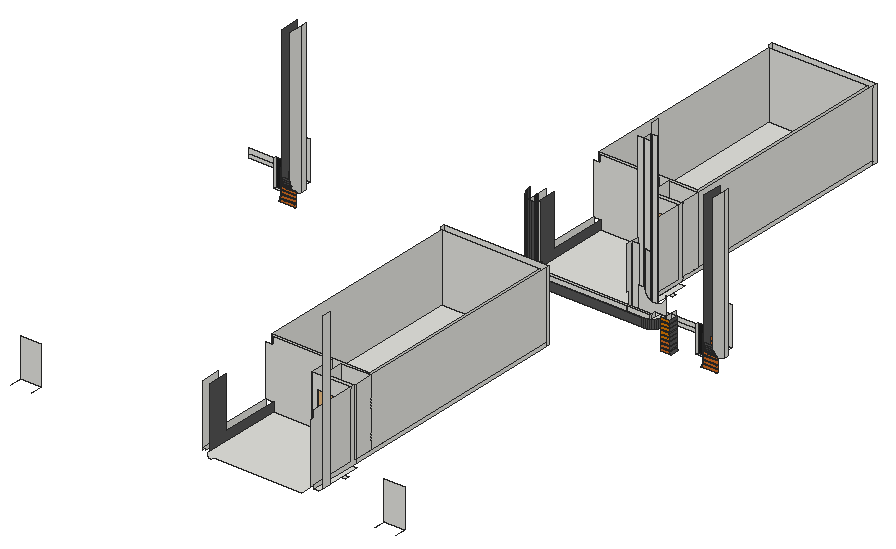
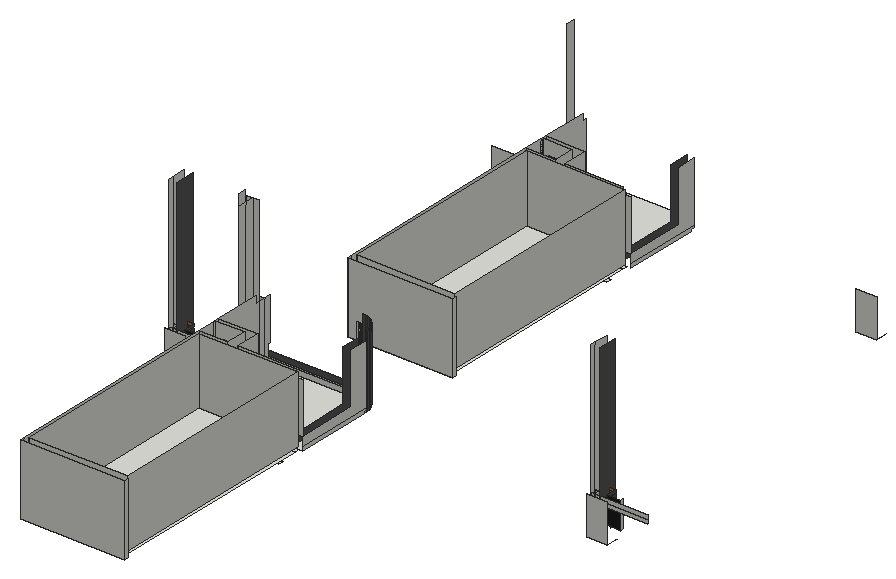
# SketchUp Ruby script. Lengths in inches.
U = 1.inch
M = Sketchup.active_model
def pt(a) = Geom::Point3d.new(a.map { |v| v * U })
def face(e, loops, mat)
  f = e.add_face(loops[0].map { |a| pt(a) })
  loops[1..].each { |l| e.add_face(l.map { |a| pt(a) }).erase! }
  f.material = f.back_material = mat if mat
  f
end
# faces: each face lists its corners as indices into pts; further lists are holes
def faces(e, pts, list, mat = nil) = list.each { |f| face(e, (f[0].is_a?(Array) ? f : [f]).map { |l| l.map { |i| pts[i] } }, mat) }
# xy, xz, yz: faces in a plane at the given z, y or x. An outline is a flat list of corners, or four numbers for a rectangle; further outlines are holes
def ring(l) = l.size == 4 ? [[l[0], l[1]], [l[2], l[1]], [l[2], l[3]], [l[0], l[3]]] : l.each_slice(2).to_a
def flat(e, list, mat, &to3) = list.each { |f| face(e, (f[0].is_a?(Array) ? f : [f]).map { |l| ring(l).map { |u, v| to3.(u, v) } }, mat) }
def xy(e, z, list, mat = nil) = flat(e, list, mat) { |x, y| [x, y, z] }
def xz(e, y, list, mat = nil) = flat(e, list, mat) { |x, z| [x, y, z] }
def yz(e, x, list, mat = nil) = flat(e, list, mat) { |y, z| [x, y, z] }
def lines(e, pts, list) = list.each { |a, b| e.add_line(pt(pts[a]), pt(pts[b])) }
# prism: a flat outline (further loops are holes) pulled along v
def prism(e, loops, v, mat = nil)
  f = face(e, loops, mat); d = Geom::Vector3d.new(v.map { |x| x * U })
  f.pushpull(f.normal.samedirection?(d) ? d.length : -d.length)
end
def box(e, o, s, mat = nil) = prism(e, [[o, [o[0] + s[0], o[1], o[2]], [o[0] + s[0], o[1] + s[1], o[2]], [o[0], o[1] + s[1], o[2]]]], [0, 0, s[2]], mat)
def at(x, y, z, deg = 0) = Geom::Transformation.translation(pt([x, y, z])) * Geom::Transformation.rotation(ORIGIN, Z_AXIS, deg.degrees)
def axes(o, x, y, z) = Geom::Transformation.new([*x, 0, *y, 0, *z, 0, *pt(o).to_a, 1])
def part(name) = M.definitions.add(name)
# library, detail: a bought-in or finely detailed component or shape, given as its bounding box
def library(name, o, s) = part(name).tap { |d| box(d.entities, o, s) }
def detail(e, o, s) = box(e.add_group.entities, o, s)
def put(e, d, t, mat = nil) = e.add_instance(d, t).tap { |i| i.material = mat if mat }
def group(e, t, mat = nil) = e.add_group.tap { |g| g.transformation = t; g.material = mat if mat }.entities
root = M.entities
M.materials.add("[0039_DarkOrange]").color = [219, 120, 0]
M.materials.add("[0041_Chocolate]").color = [210, 105, 30]
M.materials.add("[Color M06]").color = [84, 84, 84]
M.materials.add("[Color M08]").color = [30, 30, 30]
c1 = library("元件\#5",[-4.39,0,0],[5.37,35.83,90.55])
xy(root,90.875,[[1548.19,971.36,1577.46,972.36],[2230.65,971.36,2248.83,972.36],[2302.81,971.36,2332.08,972.36]],"[0041_Chocolate]")
xy(root,95.51,[[1985.87,439.98,2033.5,448.51],[2018.31,1130.875,2065.93,1139.4]])
xy(root,95.83,[[1550.05,971.36,1577.46,972.36],[2230.65,971.36,2246.96,972.36],[2304.68,971.36,2332.08,972.36]],"[0041_Chocolate]")
xy(root,97.27,[[1525.8,986.55,1550.24,991.24],[2280.42,986.55,2304.87,991.24]])
xy(root,97.9375,[[1550.33,971.36,1577.46,972.36],[2230.65,971.36,2246.69,972.36],[2304.96,971.36,2332.08,972.36]],"[0041_Chocolate]")
xy(root,101.1875,[[2078.42,397.86,2125.61,405.05],[2110.86,1088.75,2158.05,1095.9375]])
xy(root,102.89,[[1550.98,971.36,1577.46,972.36],[2230.65,971.36,2246.03,972.36],[2305.61,971.36,2332.08,972.36]],"[0041_Chocolate]")
xy(root,105,[[1550.98,971.36,1577.46,972.36],[2230.65,971.36,2246.03,972.36],[2305.61,971.36,2332.08,972.36]],"[0041_Chocolate]")
xy(root,109.9375,[[1562.99,990,1578.33,993.35],[2317.62,990,2332.96,993.35]])
xy(root,109.95,[[1550.98,971.36,1577.46,972.36],[2230.65,971.36,2246.03,972.36],[2305.61,971.36,2332.08,972.36]],"[0041_Chocolate]")
xy(root,112.0625,[[2230.65,971.36,2246.03,972.36]],"[0039_DarkOrange]")
xy(root,112.0625,[[1550.98,971.36,1577.46,972.36],[2305.61,971.36,2332.08,972.36]],"[0041_Chocolate]")
xy(root,117.02,[[2230.65,971.36,2246.03,972.36]],"[0039_DarkOrange]")
xy(root,117.02,[[1550.98,971.36,1577.46,972.36],[2305.61,971.36,2332.08,972.36]],"[0041_Chocolate]")
xy(root,119.125,[[2230.65,971.36,2246.03,972.36]],"[0039_DarkOrange]")
xy(root,119.125,[[1550.98,971.36,1577.46,972.36],[2305.61,971.36,2332.08,972.36]],"[0041_Chocolate]")
xy(root,124.08,[[2230.65,971.36,2246.03,972.36]],"[0039_DarkOrange]")
xy(root,124.08,[[1550.98,971.36,1577.46,972.36],[2305.61,971.36,2332.08,972.36]],"[0041_Chocolate]")
xy(root,126.125,[[2137,312.8125,2146.71,397.86],[2068.38,397.86,2087.21,397.86,2087.21,448.51,1957.13,448.51,1957.13,439.98,2068.38,439.98],[2087.21,397.86,2137,406.38],[2087.21,406.38,2137,830.91],[1957.13,448.51,2087.21,830.91],
  [1949.9,830.91,2137,838.14],[2012.97,958.64,2008.97,958.91,2005.04,959.6875,2002.6,960.52,2215.38,960.52,2212.34,959.49,2209.17,958.86,2205.95,958.64],[2002.6,960.52,2001.25,960.98,1997.65,962.75,1994.32,964.98,1991.31,967.62,1989.57,969.61,1988.67,970.63,1986.4375,973.96,1984.67,977.56,1983.38,981.35,1982.6,985.28,1982.33,989.28,1982.33,1130.875,2100.82,1130.875,2100.82,1088.75,2169.44,1088.75,2169.44,996.48,2179.15,996.48,2179.15,1003.71,2230.65,1003.71,2230.65,996.48,2230.15,996.48,2230.15,983.34,2230.65,983.34,2230.4375,980.12,2229.81,976.95,2228.77,973.89,2227.34,970.99,2225.54,968.31,2223.41,965.88,2220.98,963.75,2218.3,961.95,2215.4,960.52],[2230.15,983.34,2230.65,993.35],[2230.15,993.35,2230.65,996.48],
  [2169.44,996.48,2179.15,1003.71],[2169.44,1003.71,2179.15,1088.75],[2179.15,1003.71,2179.46,1012.23],[2179.46,1003.71,2181.03,1012.23],[2181.03,1003.71,2190.68,1012.23],
  [2190.68,1003.71,2230.65,1012.23],[2179.15,1012.23,2179.46,1027.17],[2179.46,1012.23,2181.03,1027.17],[2100.82,1088.75,2119.65,1088.75,2119.65,1139.4,1989.57,1139.4,1989.57,1130.875,2100.82,1130.875],[2119.65,1088.75,2169.44,1097.28],
  [2119.65,1097.28,2169.44,1521.81],[1989.57,1139.4,2119.65,1521.81],[1982.33,1521.81,2169.44,1529.04]])
xy(root,126.1875,[[2230.65,971.36,2246.03,972.36]],"[0039_DarkOrange]")
xy(root,126.1875,[[1550.98,971.36,1577.46,972.36],[2305.61,971.36,2332.08,972.36]],"[0041_Chocolate]")
xy(root,128.75,[[1982.33,985.23,1995.33,996.48]])
xy(root,131.14,[[2230.65,971.36,2246.03,972.36]],"[0039_DarkOrange]")
xy(root,131.14,[[1550.98,971.36,1577.46,972.36],[2305.61,971.36,2332.08,972.36]],"[0041_Chocolate]")
xy(root,132.47,[[1980.54,281.47,1980.54,285.84,2137,285.84,2137,395.98,2125.61,395.98,2125.61,403.17,2078.42,403.17,2078.42,395.98,2066.68,395.98,2066.68,439.98,1963.61,439.98,1963.61,298.39,1963.76,296.18,1964.1875,294.01,1964.9,291.91,1965.88,289.93,1967.11,288.09,1968.57,286.42,1970.23,284.96,1972.07,283.73,1974.06,282.75,1976.16,282.04,1978.33,281.61],[2084.26,403.17,2137,439.98],[1955.4,445.49,2131.5,825.41],[2012.97,972.36,2012.97,976.74,2169.44,976.74,2169.44,1086.875,2158.05,1086.875,2158.05,1094.0625,2110.86,1094.0625,2110.86,1086.875,2099.12,1086.875,2099.12,1130.875,1996.05,1130.875,1996.05,989.28,1996.2,987.07,1996.625,984.9,1997.34,982.81,1998.32,980.82,1999.55,978.98,2001.01,977.32,2002.67,975.86,2004.51,974.63,2006.5,973.65,2008.59,972.9375,2010.76,972.5],[2012.97,972.36,2169.44,976.74],
  [2169.44,972.36,2210.03,976.74],[2169.44,976.74,2210.03,983.34],[2169.44,983.34,2210.03,1003.71],[2116.69,1094.0625,2169.44,1130.875],[1987.84,1136.38,2163.94,1516.3]])
xy(root,133.25,[[2230.65,971.36,2246.03,972.36]],"[0039_DarkOrange]")
xy(root,133.25,[[1550.98,971.36,1577.46,972.36],[2305.61,971.36,2332.08,972.36]],"[0041_Chocolate]")
xy(root,138.2,[[2230.65,971.36,2246.03,972.36]],"[0039_DarkOrange]")
xy(root,138.2,[[1550.98,971.36,1577.46,972.36],[2305.61,971.36,2332.08,972.36]],"[0041_Chocolate]")
xy(root,140.3125,[[2230.65,971.36,2246.03,972.36]],"[0039_DarkOrange]")
xy(root,140.3125,[[1550.98,971.36,1577.46,972.36],[2305.61,971.36,2332.08,972.36]],"[0041_Chocolate]")
xz(root,343.15,[[1588.26,96.14,1624.95,165.14],[2238.76,96.14,2275.45,165.14]])
xz(root,395.98,[[2066.68,132.47,2078.42,132.47,2078.42,227.53,2125.61,227.53,2125.61,132.47,2137,132.47,2137,252.47,2066.68,252.47]])
xz(root,403.17,[[2078.42,132.47,2084.26,227.53],[2084.26,132.47,2125.61,227.53],[2125.61,132.47,2125.61,227.53,2084.26,227.53,2084.26,252.47,2137,252.47,2137,132.47]])
xz(root,439.98,[[1963.61,132.47,2066.68,132.47,2066.68,252.47,1963.61,252.47,1963.61,240.16,1949.9,240.16,1949.9,148.66,1963.61,148.66],[2084.26,132.47,2137,252.47]])
xz(root,445.49,[[1955.4,132.47,2131.5,252.47]])
xz(root,825.41,[[1955.4,132.47,2131.5,252.47]])
xz(root,838.14,[[1949.9,126.125,2137,252.47]])
xz(root,958.64,[[2012.97,126.125,2205.95,126.125,2205.95,141.26,2026.42,141.26,2024.64,141.46,2022.9,141.89,2021.22,142.53,2019.64,143.38,2018.1875,144.42,2016.87,145.64,2015.72,147.01,2014.75,148.52,2013.98,150.14,2013.43,151.84,2013.09,153.6,2012.97,155.39]],"[Color M06]")
xz(root,971.36,[[2230.65,112.0625,2246.03,117.02],[2230.65,119.125,2246.03,124.08],[2230.65,126.1875,2246.03,131.14],[2230.65,133.25,2246.03,138.2],[2230.65,140.3125,2246.03,145.27]],"[0039_DarkOrange]")
xz(root,971.36,[[1548.19,90.875,1577.46,90.875,1577.46,95.83,1550.05,95.83,1549.97,95.18],[2230.65,90.875,2248.83,90.875,2247.05,95.18,2246.96,95.83,2230.65,95.83],[2302.81,90.875,2332.08,90.875,2332.08,95.83,2304.68,95.83,2304.59,95.18],[1550.33,97.9375,1577.46,97.9375,1577.46,102.89,1550.98,102.89],[2230.65,97.9375,2246.69,97.9375,2246.03,102.89,2230.65,102.89],
  [2304.96,97.9375,2332.08,97.9375,2332.08,102.89,2305.61,102.89],[1550.98,105,1577.46,109.95],[2230.65,105,2246.03,109.95],[2305.61,105,2332.08,109.95],[1550.98,112.0625,1577.46,117.02],
  [2305.61,112.0625,2332.08,117.02],[1550.98,119.125,1577.46,124.08],[2305.61,119.125,2332.08,124.08],[1550.98,126.1875,1577.46,131.14],[2305.61,126.1875,2332.08,131.14],
  [1550.98,133.25,1577.46,138.2],[2305.61,133.25,2332.08,138.2],[1550.98,140.3125,1577.46,145.27],[2305.61,140.3125,2332.08,145.27]],"[0041_Chocolate]")
xz(root,972.36,[[2012.97,132.47,2169.44,141.26],[2169.44,132.47,2210.03,141.26]])
xz(root,972.36,[[2230.65,117.02,2246.03,119.125],[2230.65,124.08,2246.03,126.1875],[2230.65,131.14,2246.03,133.25],[2230.65,138.2,2246.03,140.3125]],"[0039_DarkOrange]")
xz(root,972.36,[[1550.05,95.83,1577.46,95.83,1577.46,97.9375,1550.33,97.9375],[2230.65,95.83,2246.96,95.83,2246.69,97.9375,2230.65,97.9375],[2304.68,95.83,2332.08,95.83,2332.08,97.9375,2304.96,97.9375],[1550.98,102.89,1577.46,105],[2230.65,102.89,2246.03,105],
  [2305.61,102.89,2332.08,105],[1550.98,109.95,1577.46,112.0625],[2230.65,109.95,2246.03,112.0625],[2305.61,109.95,2332.08,112.0625],[1550.98,117.02,1577.46,119.125],
  [2305.61,117.02,2332.08,119.125],[1550.98,124.08,1577.46,126.1875],[2305.61,124.08,2332.08,126.1875],[1550.98,131.14,1577.46,133.25],[2305.61,131.14,2332.08,133.25],
  [1550.98,138.2,1577.46,140.3125],[2305.61,138.2,2332.08,140.3125]],"[0041_Chocolate]")
xz(root,976.74,[[2012.97,132.47,2210.03,141.26]])
xz(root,983.34,[[1570.66,126.125,1571.54,141.26],[1571.54,126.125,1577.46,141.26],[2325.29,126.125,2326.17,141.26],[2326.17,126.125,2332.08,141.26],[2169.44,132.47,2181.03,240.16],
  [2181.03,132.47,2210.03,132.47,2210.03,141.26,2230.65,141.26,2230.65,174.51,2230.62,173.46,2230.54,172.42,2230.4,171.38,2230.21,170.36,2229.97,169.34,2229.67,168.33,2229.32,167.35,2228.92,166.38,2228.47,165.4375,2227.97,164.52,2227.42,163.625,2226.83,162.76,2226.19,161.93,2225.52,161.14,2224.8,160.38,2224.04,159.66,2223.24,158.98,2222.41,158.34,2221.55,157.75,2220.66,157.2,2219.74,156.7,2218.79,156.25,2217.83,155.85,2216.84,155.5,2215.84,155.21,2214.82,154.96,2213.79,154.77,2212.75,154.64,2211.71,154.55,2210.66,154.53,2209.62,154.55,2208.58,154.64,2207.54,154.77,2206.51,154.96,2205.49,155.21,2204.49,155.5,2203.5,155.85,2202.54,156.25,2201.59,156.7,2200.67,157.2,2199.78,157.75,2198.92,158.34,2198.09,158.98,2197.29,159.66,2196.53,160.38,2195.8125,161.14,2195.13,161.93,2194.5,162.76,2193.9,163.625,2193.36,164.52,2192.86,165.4375,2192.41,166.38,2192.01,167.35,2191.66,168.33,2191.36,169.34,2191.12,170.36,2190.93,171.38,2190.79,172.42,2190.71,173.46,2190.68,174.51,2181.03,174.51]])
xz(root,986.55,[[1550.24,97.27,1550.98,97.27,1550.98,102.89,1550.33,97.9375],[2304.87,97.27,2305.61,97.27,2305.61,102.89,2304.96,97.9375]])
xz(root,991.24,[[1525.8,97.27,1550.24,97.27,1550.33,97.9375,1550.98,102.89,1550.98,145.27,1525.8,145.27],[2280.42,97.27,2304.87,97.27,2304.96,97.9375,2305.61,102.89,2305.61,145.27,2280.42,145.27]],"[Color M08]")
xz(root,993.35,[[2230.15,95.62,2230.65,126.125],[1562.99,109.9375,1570.66,126.125],[1570.66,109.9375,1571.54,126.125],[1571.54,109.9375,1578.33,126.125],[2317.62,109.9375,2325.29,126.125],
  [2325.29,109.9375,2326.17,126.125],[2326.17,109.9375,2332.96,126.125],[1476.02,126.125,1562.99,132.47],[1562.99,126.125,1570.66,132.47],[1570.66,126.125,1571.54,132.47],
  [1571.54,126.125,1578.33,132.47],[2230.65,126.125,2317.62,132.47],[2317.62,126.125,2325.29,132.47],[2325.29,126.125,2326.17,132.47],[2326.17,126.125,2332.96,132.47],
  [1476.02,132.47,1562.99,141.26],[1562.99,132.47,1570.66,141.26],[1570.66,132.47,1571.54,141.26],[1571.54,132.47,1578.33,141.26],[2230.65,132.47,2317.62,141.26],
  [2317.62,132.47,2325.29,141.26],[2325.29,132.47,2326.17,141.26],[2326.17,132.47,2332.96,141.26]])
xz(root,996.48,[[2169.44,126.125,2179.15,402.64],[2179.15,126.125,2181.03,126.125,2181.03,226.8,2190.68,226.8,2190.68,402.64,2179.15,402.64]])
xz(root,1003.71,[[2169.44,126.125,2230.65,132.47]])
xz(root,1012.23,[[2179.15,126.125,2181.03,402.64],[2181.03,126.125,2190.68,402.64]])
xz(root,1034.04,[[1516.57,96.14,1553.26,165.14],[2271.2,96.14,2307.88,165.14]])
xz(root,1086.875,[[2099.12,132.47,2110.86,132.47,2110.86,227.53,2158.05,227.53,2158.05,132.47,2169.44,132.47,2169.44,252.47,2099.12,252.47]])
xz(root,1094.0625,[[2110.86,132.47,2116.69,227.53],[2116.69,132.47,2158.05,227.53],[2158.05,132.47,2158.05,227.53,2116.69,227.53,2116.69,252.47,2169.44,252.47,2169.44,132.47]])
xz(root,1130.875,[[1996.05,132.47,2099.12,132.47,2099.12,252.47,1996.05,252.47,1996.05,240.16,1982.33,240.16,1982.33,148.66,1996.05,148.66],[2116.69,132.47,2169.44,252.47]])
xz(root,1136.38,[[1987.84,132.47,2163.94,252.47]])
xz(root,1516.3,[[1987.84,132.47,2163.94,252.47]])
xz(root,1529.04,[[1982.33,126.125,2169.44,252.47]])
yz(root,1525.8,[[986.55,97.27,991.24,145.27]])
yz(root,1550.98,[[972.36,102.89,991.24,105],[971.36,105,991.24,109.95],[972.36,109.95,991.24,112.0625],[971.36,112.0625,991.24,117.02],[972.36,117.02,991.24,119.125],
  [971.36,119.125,991.24,124.08],[972.36,124.08,991.24,126.1875],[971.36,126.1875,991.24,131.14],[972.36,131.14,991.24,133.25],[971.36,133.25,991.24,138.2],
  [972.36,138.2,991.24,140.3125],[971.36,140.3125,991.24,145.27]],"[Color M06]")
yz(root,1562.99,[[990,109.9375,985.91,110.21,981.89,111.01,978,112.32,974.32,114.14,970.91,116.42,967.83,119.12,965.125,122.21,962.85,125.62,961.03,129.3,959.71,133.18,958.91,137.2,958.64,141.3,958.64,376.875,993.35,376.875,993.35,109.9375]],"[Color M06]")
yz(root,1570.66,[[983.34,126.125,993.35,141.26]])
yz(root,1578.33,[[990,109.9375,993.35,109.9375,993.35,376.875,983.34,376.875,983.34,110.72,985.91,110.21],[983.34,110.72,983.34,376.875,958.64,376.875,958.64,141.3,958.91,137.2,959.71,133.18,961.03,129.3,962.85,125.62,965.125,122.21,967.83,119.12,970.91,116.42,974.32,114.14,978,112.32,981.89,111.01]])
yz(root,1949.9,[[305.58,126.125,305.58,128.75,298.39,128.75,298.39,132.47,439.98,132.47,439.98,126.125],[830.91,126.125,838.14,252.47],[298.39,132.47,298.39,240.16,333.33,240.16,333.33,148.66,439.98,148.66,439.98,132.47]])
yz(root,1955.4,[[445.49,132.47,825.41,252.47]])
yz(root,1963.61,[[298.39,132.47,439.98,132.47,439.98,148.66,333.33,148.66,333.33,240.16,298.39,240.16]],"[Color M06]")
yz(root,1982.33,[[989.28,126.125,996.48,128.75],[996.48,126.125,996.48,128.75,989.28,128.75,989.28,132.47,1130.875,132.47,1130.875,126.125],[1521.81,126.125,1529.04,252.47],[989.28,132.47,989.28,240.16,1024.22,240.16,1024.22,148.66,1130.875,148.66,1130.875,132.47]])
yz(root,1987.84,[[1136.38,132.47,1516.3,252.47]])
yz(root,1996.05,[[989.28,132.47,1130.875,132.47,1130.875,148.66,1024.22,148.66,1024.22,240.16,989.28,240.16]],"[Color M06]")
yz(root,2012.97,[[972.36,132.47,976.74,155.39]])
yz(root,2066.68,[[395.98,132.47,439.98,252.47]])
yz(root,2078.42,[[395.98,132.47,403.17,227.53]])
yz(root,2084.26,[[403.17,132.47,439.98,252.47]])
yz(root,2099.12,[[1086.875,132.47,1130.875,252.47]])
yz(root,2110.86,[[1086.875,132.47,1094.0625,227.53]])
yz(root,2116.69,[[1094.0625,132.47,1130.875,252.47]])
yz(root,2125.61,[[395.98,132.47,403.17,227.53]])
yz(root,2131.5,[[445.49,132.47,825.41,252.47]])
yz(root,2137,[[312.8125,126.125,312.8125,132.47,395.98,132.47,395.98,252.47,403.17,252.47,403.17,132.47,406.38,132.47,406.38,126.125],[406.38,126.125,830.91,132.47],[830.91,126.125,838.14,252.47],[305.58,132.47,305.58,240.16,312.8125,240.16,312.8125,252.47,395.98,252.47,395.98,132.47],[403.17,132.47,406.38,252.47],
  [406.38,132.47,439.98,252.47],[439.98,132.47,830.91,252.47]])
yz(root,2146.71,[[321.34,126.125,337.5625,402.64]])
yz(root,2158.05,[[1086.875,132.47,1094.0625,227.53]])
yz(root,2163.94,[[1136.38,132.47,1516.3,252.47]])
yz(root,2169.44,[[1003.71,126.125,1003.71,132.47,1086.875,132.47,1086.875,252.47,1094.0625,252.47,1094.0625,132.47,1097.28,132.47,1097.28,126.125],[1097.28,126.125,1521.81,132.47],[1521.81,126.125,1529.04,252.47],[972.36,132.47,972.36,141.26,976.74,141.26,976.74,163.7,972.36,163.7,972.36,240.16,983.34,240.16,983.34,132.47],[983.34,132.47,996.48,240.16],
  [996.48,132.47,996.48,240.16,1003.71,240.16,1003.71,252.47,1086.875,252.47,1086.875,132.47],[1094.0625,132.47,1097.28,252.47],[1097.28,132.47,1130.875,252.47],[1130.875,132.47,1521.81,252.47]])
yz(root,2179.15,[[996.48,126.125,1012.23,402.64],[1012.23,126.125,1028.46,402.64]])
yz(root,2181.03,[[1012.23,126.125,1027.17,421.25]])
yz(root,2210.03,[[972.36,132.47,976.74,141.26],[976.74,132.47,983.34,141.26]])
yz(root,2230.15,[[993.35,95.62,996.48,126.125]])
yz(root,2230.65,[[983.34,126.125,993.35,141.26],[993.35,126.125,996.48,132.47],[996.48,126.125,1003.71,132.47],[993.35,132.47,996.48,141.26],[996.48,132.47,1003.71,141.26]])
yz(root,2246.03,[[972.36,102.89,986.55,105],[971.36,105,986.55,109.95],[972.36,109.95,986.55,112.0625],[971.36,112.0625,986.55,117.02],[972.36,117.02,986.55,119.125],
  [971.36,119.125,986.55,124.08],[972.36,124.08,986.55,126.1875],[971.36,126.1875,986.55,131.14],[972.36,131.14,986.55,133.25],[971.36,133.25,986.55,138.2],
  [972.36,138.2,986.55,140.3125],[971.36,140.3125,986.55,145.27]],"[Color M06]")
yz(root,2280.42,[[986.55,97.27,991.24,145.27]])
yz(root,2305.61,[[972.36,102.89,991.24,105],[971.36,105,991.24,109.95],[972.36,109.95,991.24,112.0625],[971.36,112.0625,991.24,117.02],[972.36,117.02,991.24,119.125],
  [971.36,119.125,991.24,124.08],[972.36,124.08,991.24,126.1875],[971.36,126.1875,991.24,131.14],[972.36,131.14,991.24,133.25],[971.36,133.25,991.24,138.2],
  [972.36,138.2,991.24,140.3125],[971.36,140.3125,991.24,145.27]],"[Color M06]")
yz(root,2317.62,[[990,109.9375,985.91,110.21,981.89,111.01,978,112.32,974.32,114.14,970.91,116.42,967.83,119.12,965.125,122.21,962.85,125.62,961.03,129.3,959.71,133.18,958.91,137.2,958.64,141.3,958.64,376.875,993.35,376.875,993.35,109.9375]],"[Color M06]")
yz(root,2325.29,[[983.34,126.125,993.35,141.26]])
yz(root,2332.96,[[990,109.9375,993.35,109.9375,993.35,376.875,983.34,376.875,983.34,110.72,985.91,110.21],[983.34,110.72,983.34,376.875,958.64,376.875,958.64,141.3,958.91,137.2,959.71,133.18,961.03,129.3,962.85,125.62,965.125,122.21,967.83,119.12,970.91,116.42,974.32,114.14,978,112.32,981.89,111.01]])
p = [[1548.19,986.55,90.875],[1548.19,972.36,90.875],[1548.19,971.36,90.875],[1549.97,971.36,95.18],[1549.97,986.55,95.18],[2247.05,986.55,95.18],
  [2247.05,971.36,95.18],[2248.83,971.36,90.875],[2248.83,972.36,90.875],[2248.83,986.55,90.875],[2302.81,986.55,90.875],[2302.81,972.36,90.875],
  [2302.81,971.36,90.875],[2304.59,971.36,95.18],[2304.59,986.55,95.18],[1550.05,971.36,95.83],[1550.05,972.36,95.83],[1550.05,986.55,95.83],
  [2246.96,986.55,95.83],[2246.96,972.36,95.83],[2246.96,971.36,95.83],[2304.68,971.36,95.83],[2304.68,972.36,95.83],[2304.68,986.55,95.83],
  [1550.33,972.36,97.9375],[1550.33,986.55,97.9375],[1550.24,986.55,97.27],[2246.69,972.36,97.9375],[2246.69,986.55,97.9375],[2304.96,972.36,97.9375],
  [2304.96,986.55,97.9375],[2304.87,986.55,97.27],[1550.33,991.24,97.9375],[1550.24,991.24,97.27],[2304.96,991.24,97.9375],[2304.87,991.24,97.27],
  [1550.33,971.36,97.9375],[1550.98,971.36,102.89],[1550.98,972.36,102.89],[1550.98,986.55,102.89],[2246.03,986.55,102.89],[2246.03,972.36,102.89],
  [2246.03,971.36,102.89],[2246.69,971.36,97.9375],[2304.96,971.36,97.9375],[2305.61,971.36,102.89],[2305.61,972.36,102.89],[2305.61,986.55,102.89],
  [1550.98,991.24,102.89],[2305.61,991.24,102.89],[1578.33,990,109.9375],[1578.33,985.91,110.21],[1562.99,985.91,110.21],[1562.99,990,109.9375],
  [2332.96,990,109.9375],[2332.96,985.91,110.21],[2317.62,985.91,110.21],[2317.62,990,109.9375],[1578.33,983.34,110.72],[1578.33,981.89,111.01],
  [1562.99,981.89,111.01],[2332.96,983.34,110.72],[2332.96,981.89,111.01],[2317.62,981.89,111.01],[1578.33,978,112.32],[1562.99,978,112.32],
  [2332.96,978,112.32],[2317.62,978,112.32],[1578.33,974.32,114.14],[1562.99,974.32,114.14],[2332.96,974.32,114.14],[2317.62,974.32,114.14],
  [1578.33,970.91,116.42],[1562.99,970.91,116.42],[2332.96,970.91,116.42],[2317.62,970.91,116.42],[1578.33,967.83,119.12],[1562.99,967.83,119.12],
  [2332.96,967.83,119.12],[2317.62,967.83,119.12],[1578.33,965.125,122.21],[1562.99,965.125,122.21],[2332.96,965.125,122.21],[2317.62,965.125,122.21],
  [1578.33,962.85,125.62],[1562.99,962.85,125.62],[2332.96,962.85,125.62],[2317.62,962.85,125.62],[1578.33,961.03,129.3],[1562.99,961.03,129.3],
  [2332.96,961.03,129.3],[2317.62,961.03,129.3],[2012.97,958.64,258.13],[2008.97,958.91,258.13],[2008.97,958.91,126.125],[2012.97,958.64,126.125],
  [2012.97,958.64,155.39],[2012.97,958.64,164.97],[2012.97,958.64,240.16],[2209.17,958.86,141.26],[2205.95,958.64,141.26],[2205.95,958.64,126.125],
  [2209.17,958.86,126.125],[2005.04,959.6875,258.13],[2005.04,959.6875,126.125],[2212.34,959.49,141.26],[2212.34,959.49,126.125],[2215.4,960.52,141.26],
  [2215.38,960.52,126.125],[2215.4,960.52,126.125],[2001.25,960.98,258.13],[2001.25,960.98,126.125],[2002.6,960.52,126.125],[2218.3,961.95,141.26],
  [2218.3,961.95,126.125],[1997.65,962.75,258.13],[1997.65,962.75,126.125],[2220.98,963.75,141.26],[2220.98,963.75,126.125],[1994.32,964.98,258.13],
  [1994.32,964.98,126.125],[2223.41,965.88,141.26],[2223.41,965.88,126.125],[1991.31,967.62,258.13],[1991.31,967.62,126.125],[2225.54,968.31,141.26],
  [2225.54,968.31,126.125],[1988.67,970.63,258.13],[1988.67,970.63,126.125],[1989.57,969.61,126.125],[2227.34,970.99,141.26],[2227.34,970.99,126.125],
  [1986.4375,973.96,258.13],[1986.4375,973.96,126.125],[2228.01,972.36,141.26],[2228.77,973.89,126.125],[2228.77,973.89,141.26],[2229.81,976.95,141.26],
  [2229.81,976.95,126.125],[1984.67,977.56,258.13],[1984.67,977.56,126.125],[2230.4375,980.12,141.26],[2230.4375,980.12,126.125],[1983.38,981.35,258.13],
  [1983.38,981.35,126.125],[2230.65,983.34,141.26],[2230.65,983.34,126.125],[1982.6,985.28,258.13],[1982.6,985.28,126.125],[1982.33,989.28,240.16],
  [1982.33,989.28,132.47],[1982.33,989.28,128.75],[1982.33,989.28,126.125],[1982.33,989.28,258.13],[1578.33,959.71,133.18],[1562.99,959.71,133.18],
  [2332.96,959.71,133.18],[2317.62,959.71,133.18],[2010.76,972.5,252.47],[2012.97,972.36,252.47],[2012.97,972.36,240.16],[2012.97,972.36,164.97],
  [2012.97,972.36,163.7],[2012.97,972.36,155.39],[2012.97,972.36,141.26],[2012.97,972.36,132.47],[2010.76,972.5,132.47],[2008.59,972.9375,252.47],
  [2008.59,972.9375,132.47],[2006.5,973.65,252.47],[2006.5,973.65,132.47],[2004.51,974.63,252.47],[2004.51,974.63,132.47],[2002.67,975.86,252.47],
  [2002.67,975.86,132.47],[2001.01,977.32,252.47],[2001.01,977.32,132.47],[1999.55,978.98,252.47],[1999.55,978.98,132.47],[1998.32,980.82,252.47],
  [1998.32,980.82,132.47],[1997.34,982.81,252.47],[1997.34,982.81,132.47],[1996.625,984.9,252.47],[1996.625,984.9,132.47],[1996.2,987.07,252.47],
  [1996.2,987.07,132.47],[1996.05,989.28,252.47],[1996.05,989.28,132.47],[1996.05,989.28,240.16],[1578.33,958.91,137.2],[1562.99,958.91,137.2],
  [2332.96,958.91,137.2],[2317.62,958.91,137.2],[1578.33,958.64,141.3],[1562.99,958.64,141.3],[2332.96,958.64,141.3],[2317.62,958.64,141.3],
  [1624.95,321.34,96.14],[1624.95,343.15,96.14],[1588.26,321.34,96.14],[1588.26,343.15,96.14],[2275.45,321.34,96.14],[2275.45,343.15,96.14],
  [2238.76,321.34,96.14],[2238.76,343.15,96.14],[1553.26,1012.23,96.14],[1553.26,1034.04,96.14],[1516.57,1012.23,96.14],[1516.57,1034.04,96.14],
  [2271.2,1012.23,96.14],[2271.2,1034.04,96.14],[2307.88,1012.23,96.14],[2307.88,1034.04,96.14]]
faces(root,p,[[0,1,2,3,4],[5,6,7,8,9],[10,11,12,13,14],[4,3,15,16,17],[18,19,20,6,5],[14,13,21,22,23],[16,24,25,26,17],[27,19,18,28],
  [22,29,30,31,23],[25,24,36,37,38,39],[40,41,42,43,27,28],[30,29,44,45,46,47],[25,39,48,32],[30,47,49,34],[50,51,52,53],[54,55,56,57],
  [58,59,60,52,51],[61,62,63,56,55],[59,64,65,60],[62,66,67,63],[64,68,69,65],[66,70,71,67],[68,72,73,69],[70,74,75,71],
  [72,76,77,73],[74,78,79,75],[76,80,81,77],[78,82,83,79],[80,84,85,81],[82,86,87,83],[84,88,89,85],[86,90,91,87],
  [92,93,94,95,96,97,98],[99,100,101,102],[93,103,104,94],[105,99,102,106],[107,105,106,108,109],[110,111,112,104,103],[113,107,109,114],[115,116,111,110],
  [117,113,114,118],[119,120,116,115],[121,117,118,122],[123,124,120,119],[125,121,122,126],[127,128,129,124,123],[130,125,126,131],[132,133,128,127],
  [134,130,131,135,136],[137,136,135,138],[139,140,133,132],[141,137,138,142],[143,144,140,139],[145,141,142,146],[147,148,144,143],[149,150,151,152,148,147,153],
  [88,154,155,89],[90,156,157,91],[154,190,191,155],[156,192,193,157],[190,194,195,191],[192,196,197,193]],"[Color M06]")
faces(root,p,[[26,25,32,33],[31,30,34,35],[158,159,160,161,162,163,164,165,166],[167,158,166,168],[169,167,168,170],[171,169,170,172],[173,171,172,174],[175,173,174,176],
  [177,175,176,178],[179,177,178,180],[181,179,180,182],[183,181,182,184],[185,183,184,186],[187,185,186,188,189]])
lines(root,p,[[198,199],[200,201],[202,203],[204,205],[206,207],[208,209],[210,211],[212,213]])
put(root,c1,axes([2078.42,396.14,132.47],[0,-1.05,0],[1.302,0,0],[0,0,1.05]))
put(root,c1,axes([2110.86,1087.03,132.47],[0,-1.05,0],[1.302,0,0],[0,0,1.05]))
